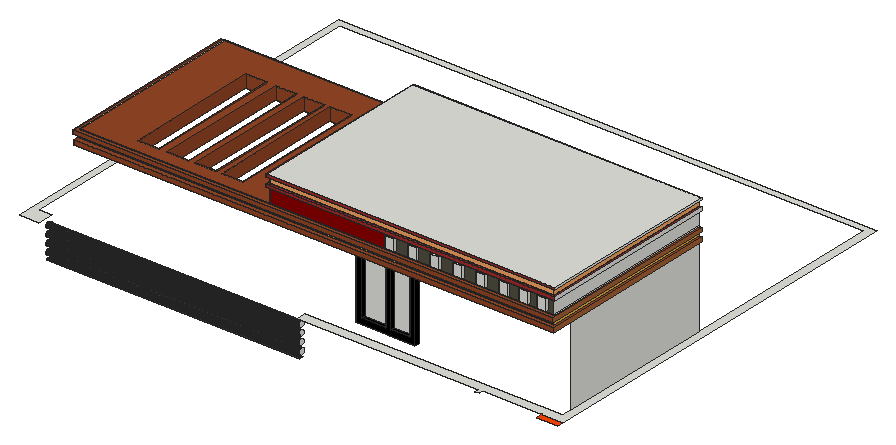
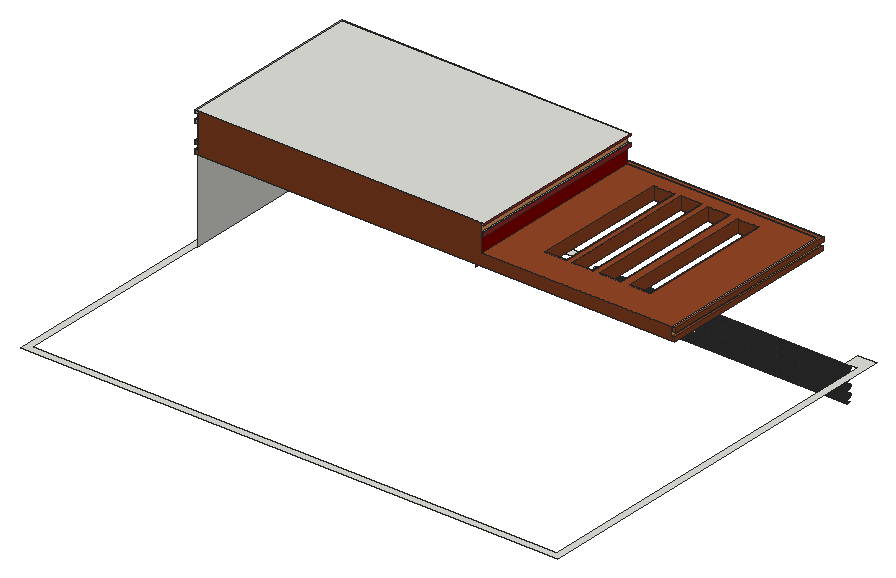
# SketchUp Ruby script. Lengths in inches.
U = 1.inch
M = Sketchup.active_model
def pt(a) = Geom::Point3d.new(a.map { |v| v * U })
def face(e, loops, mat)
  f = e.add_face(loops[0].map { |a| pt(a) })
  loops[1..].each { |l| e.add_face(l.map { |a| pt(a) }).erase! }
  f.material = f.back_material = mat if mat
  f
end
# faces: each face lists its corners as indices into pts; further lists are holes
def faces(e, pts, list, mat = nil) = list.each { |f| face(e, (f[0].is_a?(Array) ? f : [f]).map { |l| l.map { |i| pts[i] } }, mat) }
# xy, xz, yz: faces in a plane at the given z, y or x. An outline is a flat list of corners, or four numbers for a rectangle; further outlines are holes
def ring(l) = l.size == 4 ? [[l[0], l[1]], [l[2], l[1]], [l[2], l[3]], [l[0], l[3]]] : l.each_slice(2).to_a
def flat(e, list, mat, &to3) = list.each { |f| face(e, (f[0].is_a?(Array) ? f : [f]).map { |l| ring(l).map { |u, v| to3.(u, v) } }, mat) }
def xy(e, z, list, mat = nil) = flat(e, list, mat) { |x, y| [x, y, z] }
def xz(e, y, list, mat = nil) = flat(e, list, mat) { |x, z| [x, y, z] }
def yz(e, x, list, mat = nil) = flat(e, list, mat) { |y, z| [x, y, z] }
def lines(e, pts, list) = list.each { |a, b| e.add_line(pt(pts[a]), pt(pts[b])) }
# prism: a flat outline (further loops are holes) pulled along v
def prism(e, loops, v, mat = nil)
  f = face(e, loops, mat); d = Geom::Vector3d.new(v.map { |x| x * U })
  f.pushpull(f.normal.samedirection?(d) ? d.length : -d.length)
end
def box(e, o, s, mat = nil) = prism(e, [[o, [o[0] + s[0], o[1], o[2]], [o[0] + s[0], o[1] + s[1], o[2]], [o[0], o[1] + s[1], o[2]]]], [0, 0, s[2]], mat)
def at(x, y, z, deg = 0) = Geom::Transformation.translation(pt([x, y, z])) * Geom::Transformation.rotation(ORIGIN, Z_AXIS, deg.degrees)
def axes(o, x, y, z) = Geom::Transformation.new([*x, 0, *y, 0, *z, 0, *pt(o).to_a, 1])
def part(name) = M.definitions.add(name)
# library, detail: a bought-in or finely detailed component or shape, given as its bounding box
def library(name, o, s) = part(name).tap { |d| box(d.entities, o, s) }
def detail(e, o, s) = box(e.add_group.entities, o, s)
def put(e, d, t, mat = nil) = e.add_instance(d, t).tap { |i| i.material = mat if mat }
def group(e, t, mat = nil) = e.add_group.tap { |g| g.transformation = t; g.material = mat if mat }.entities
root = M.entities
M.materials.add("[0018_Brown]").color = [165, 42, 42]
M.materials.add("[0020_Red]").color = [255, 0, 0]
M.materials.add("[0021_DarkRed]").color = [139, 0, 0]
M.materials.add("[0024_OrangeRed]").color = [255, 69, 0]
M.materials.add("[0035_Tan]").color = [232, 181, 59]
M.materials.add("[0037_SandyBrown]").color = [244, 164, 96]
M.materials.add("[0137_Black]").color = [0, 0, 0]
M.materials.add("[Asphalt New]").color = [67, 60, 62]
M.materials.add("[Stone Coursed Rough]1").color = [81, 79, 64]
M.materials.add("[Wood Veneer 01]").color = [147, 70, 37]
M.materials.add("[Wood Veneer 01]1").color = [165, 96, 51]
xy(root,437.16,[[408.85,294.98,489.23,300.98]],"[0137_Black]")
xy(root,444.75,[[416.4375,294.98,449.04,300.98],[455.68,294.98,481.64,300.98]],"[0137_Black]")
xy(root,450,[[0,236.25,25.71,236.25,25.71,257.25,9,257.25,9,767.8125,720.125,767.8125,720.125,257.25,369.99,257.25,369.99,245.125,615.29,245.125,615.29,239.125,621.57,239.125,621.57,245.125,730.1875,245.125,730.1875,776.8125,0,776.8125]])
xy(root,450,[[701.81,236.125,730.1875,245.125]],"[0024_OrangeRed]")
xy(root,528.07,[[416.4375,294.98,449.04,300.98],[455.68,294.98,481.64,300.98]],"[0137_Black]")
xy(root,535.66,[[408.85,294.98,489.23,300.98]],"[0137_Black]")
xy(root,561.0625,[[706.26,270.98,706.26,294.98,507.58,294.98,507.58,300.98,720.125,300.98,720.125,270.98],[99.47,293.9,132.15,300.98],[99.47,300.98,132.15,318.33]])
xy(root,561.0625,[[[72.09,236.23,72.09,488.35,342.3125,488.35,342.3125,300.98,507.58,300.98,507.58,294.98,706.26,294.98,706.26,270.98,720.125,270.98,720.125,488.35,724.125,488.35,724.125,236.23],[253.17,261.42,281.98,445.86],[217.23,261.42,246.04,445.86],[179.29,261.42,208.11,445.86],[138.98,261.42,167.79,445.86],[99.47,293.9,132.15,318.33]]],"[Wood Veneer 01]")
xy(root,567.18,[[72.09,236.23,724.125,236.23,724.125,488.35,720.125,488.35,720.125,242.23,75.53,242.23,75.53,488.35,72.09,488.35]],"[Wood Veneer 01]")
xy(root,573.3,[[71.28,236.23,71.28,488.35,75.53,488.35,75.53,242.23,720.125,242.23,720.125,488.35,723.75,488.35,723.75,236.23]],"[Wood Veneer 01]")
xy(root,578.4375,[[71.28,236.23,723.75,236.23,723.75,488.35,720.125,488.35,720.125,242.23,75.53,242.23,75.53,488.35,71.28,488.35],[[75.53,242.23,333.59,488.35],[179.29,261.42,208.11,445.86],[217.23,261.42,246.04,445.86],[253.17,261.42,281.98,445.86],[138.98,261.42,167.79,445.86]]],"[Wood Veneer 01]")
xy(root,581.12,[[492.41,239.23,504.66,242.23],[523.34,239.23,535.59,242.23],[554.28,239.23,566.53,242.23],[585.22,239.23,597.47,242.23],[616.16,239.23,628.41,242.23],
  [647.09,239.23,659.34,242.23],[674.53,239.23,686.78,242.23],[698.84,239.23,711.09,242.23]])
xy(root,596.49,[[492.41,239.23,504.66,242.23],[523.34,239.23,535.59,242.23],[554.28,239.23,566.53,242.23],[585.22,239.23,597.47,242.23],[616.16,239.23,628.41,242.23],
  [647.09,239.23,659.34,242.23],[674.53,239.23,686.78,242.23],[698.84,239.23,711.09,242.23]])
xy(root,598.8125,[[330.96,239.23,330.96,488.35,333.59,488.35,333.59,242.23,720.125,242.23,720.125,488.35,724.125,488.35,724.125,239.23]],"[0018_Brown]")
xy(root,603.39,[[330.96,239.23,724.125,239.23,724.125,488.35,720.125,488.35,720.125,242.23,333.59,242.23,333.59,488.35,330.96,488.35]],"[0018_Brown]")
xy(root,611.61,[[330.96,239.23,330.96,488.35,333.59,488.35,333.59,242.23,720.125,242.23,720.125,488.35,723.625,488.35,723.625,239.23]],"[0018_Brown]")
xy(root,614.4375,[[330.96,239.23,723.625,488.35]])
xz(root,236.23,[[72.09,561.0625,724.125,567.18],[71.28,573.3,723.75,578.4375]],"[Wood Veneer 01]")
xz(root,239.23,[[492.41,581.12,504.66,596.49],[523.34,581.12,535.59,596.49],[554.28,581.12,566.53,596.49],[585.22,581.12,597.47,596.49],[616.16,581.12,628.41,596.49],
  [647.09,581.12,659.34,596.49],[674.53,581.12,686.78,596.49],[698.84,581.12,711.09,596.49]])
xz(root,239.23,[[330.96,598.8125,724.125,603.39],[330.96,611.61,723.625,614.4375]],"[0018_Brown]")
xz(root,242.23,[[75.53,573.3,720.125,578.4375],[333.59,598.8125,720.125,603.39]])
xz(root,242.23,[[333.59,578.4375,491.23,598.8125]],"[0021_DarkRed]")
xz(root,242.23,[[75.53,567.18,720.125,573.3]],"[0035_Tan]")
xz(root,242.23,[[333.59,603.39,720.125,611.61]],"[0037_SandyBrown]")
xz(root,242.23,[[[491.23,578.4375,720.125,598.8125],[698.84,581.12,711.09,596.49],[674.53,581.12,686.78,596.49],[647.09,581.12,659.34,596.49],[616.16,581.12,628.41,596.49],[585.22,581.12,597.47,596.49],[554.28,581.12,566.53,596.49],[523.34,581.12,535.59,596.49],[492.41,581.12,504.66,596.49]]],"[Stone Coursed Rough]1")
xz(root,261.42,[[138.98,561.0625,167.79,578.4375],[179.29,561.0625,208.11,578.4375],[217.23,561.0625,246.04,578.4375],[253.17,561.0625,281.98,578.4375]],"[Wood Veneer 01]")
xz(root,294.98,[[[408.85,437.16,489.23,535.66],[416.4375,444.75,449.04,528.07],[455.68,444.75,481.64,528.07]]],"[0137_Black]")
xz(root,300.98,[[416.4375,444.75,449.04,528.07],[455.68,444.75,481.64,528.07]])
xz(root,445.86,[[138.98,561.0625,167.79,578.4375],[179.29,561.0625,208.11,578.4375],[217.23,561.0625,246.04,578.4375],[253.17,561.0625,281.98,578.4375]],"[Wood Veneer 01]")
xz(root,488.35,[[330.96,598.8125,333.59,603.39],[720.125,598.8125,724.125,603.39],[330.96,611.61,333.59,614.4375],[720.125,611.61,723.625,614.4375]])
xz(root,488.35,[[75.53,561.0625,75.53,578.4375,333.59,578.4375,333.59,614.4375,720.125,614.4375,720.125,561.0625]],"[Wood Veneer 01]")
xz(root,488.35,[[72.09,561.0625,75.53,567.18],[720.125,561.0625,724.125,567.18],[71.28,573.3,75.53,578.4375],[720.125,573.3,723.75,578.4375]],"[Wood Veneer 01]1")
yz(root,71.28,[[236.23,573.3,488.35,578.4375]],"[Wood Veneer 01]")
yz(root,72.09,[[236.23,561.0625,488.35,567.18]],"[Wood Veneer 01]")
yz(root,75.53,[[242.23,573.3,488.35,578.4375]])
yz(root,75.53,[[242.23,567.18,488.35,573.3]],"[0035_Tan]")
yz(root,99.47,[[300.98,561.0625,318.33,562.9375]])
yz(root,138.98,[[261.42,561.0625,445.86,578.4375]],"[Wood Veneer 01]")
yz(root,167.79,[[261.42,561.0625,445.86,578.4375]],"[Wood Veneer 01]")
yz(root,179.29,[[261.42,561.0625,445.86,578.4375]],"[Wood Veneer 01]")
yz(root,208.11,[[261.42,561.0625,445.86,578.4375]],"[Wood Veneer 01]")
yz(root,217.23,[[261.42,561.0625,445.86,578.4375]],"[Wood Veneer 01]")
yz(root,246.04,[[261.42,561.0625,445.86,578.4375]],"[Wood Veneer 01]")
yz(root,253.17,[[261.42,561.0625,445.86,578.4375]],"[Wood Veneer 01]")
yz(root,281.98,[[261.42,561.0625,445.86,578.4375]],"[Wood Veneer 01]")
yz(root,330.96,[[239.23,598.8125,488.35,603.39],[239.23,611.61,488.35,614.4375]],"[0018_Brown]")
yz(root,333.59,[[242.23,598.8125,488.35,603.39]])
yz(root,333.59,[[242.23,578.4375,488.35,598.8125]],"[0021_DarkRed]")
yz(root,333.59,[[242.23,603.39,488.35,611.61]],"[0037_SandyBrown]")
yz(root,342.3125,[[300.98,557.75,488.35,561.0625]],"[0020_Red]")
yz(root,369.99,[[251.48,414.82,252.42,414.95,253.3,415.31,254.05,415.89,254.62,416.64,254.98,417.51,255.11,418.45,254.98,419.39,254.62,420.26,254.05,421.01,253.3,421.59,252.42,421.95,251.48,422.07,250.54,421.95,249.67,421.59,248.92,421.01,248.34,420.26,248.25,420.04,248.25,416.86,248.34,416.64,248.92,415.89,249.67,415.31,250.54,414.95],[248.25,416.86,247.98,417.51,247.86,418.45,247.98,419.39,248.25,420.04],[251.48,425.76,252.42,425.89,253.3,426.25,254.05,426.82,254.62,427.57,254.98,428.45,255.11,429.39,254.98,430.33,254.62,431.2,254.05,431.95,253.3,432.53,252.42,432.89,251.48,433.01,250.54,432.89,249.67,432.53,248.92,431.95,248.34,431.2,248.25,430.97,248.25,427.8,248.34,427.57,248.92,426.82,249.67,426.25,250.54,425.89],[248.25,427.8,247.98,428.45,247.86,429.39,247.98,430.33,248.25,430.97],[251.48,436.7,252.42,436.82,253.3,437.19,254.05,437.76,254.62,438.51,254.98,439.39,255.11,440.32,254.98,441.26,254.62,442.14,254.05,442.89,253.3,443.46,252.42,443.83,251.48,443.95,250.54,443.83,249.67,443.46,248.92,442.89,248.34,442.14,248.25,441.91,248.25,438.74,248.34,438.51,248.92,437.76,249.67,437.19,250.54,436.82],
  [248.25,438.74,247.98,439.39,247.86,440.32,247.98,441.26,248.25,441.91]])
yz(root,370.39,[[251.48,403.89,252.42,404.01,253.3,404.37,254.05,404.95,254.62,405.7,254.98,406.57,255.11,407.51,254.98,408.45,254.62,409.32,254.05,410.08,253.3,410.65,252.42,411.01,251.48,411.14,250.54,411.01,249.67,410.65,248.92,410.08,248.34,409.32,247.98,408.45,247.86,407.51,247.98,406.57,248.34,405.7,248.92,404.95,249.67,404.37,250.54,404.01]])
yz(root,408.85,[[294.98,437.16,300.98,535.66]],"[0137_Black]")
yz(root,416.4375,[[294.98,444.75,300.98,528.07]],"[0137_Black]")
yz(root,449.04,[[294.98,444.75,300.98,528.07]],"[0137_Black]")
yz(root,455.68,[[294.98,444.75,300.98,528.07]],"[0137_Black]")
yz(root,481.64,[[294.98,444.75,300.98,528.07]],"[0137_Black]")
yz(root,489.23,[[294.98,437.16,300.98,535.66]],"[0137_Black]")
yz(root,492.41,[[239.23,581.12,242.23,596.49]])
yz(root,504.66,[[239.23,581.12,242.23,596.49]])
yz(root,523.34,[[239.23,581.12,242.23,596.49]])
yz(root,535.59,[[239.23,581.12,242.23,596.49]])
yz(root,554.28,[[239.23,581.12,242.23,596.49]])
yz(root,566.53,[[239.23,581.12,242.23,596.49]])
yz(root,585.22,[[239.23,581.12,242.23,596.49]])
yz(root,597.47,[[239.23,581.12,242.23,596.49]])
yz(root,616.16,[[239.23,581.12,242.23,596.49]])
yz(root,628.41,[[239.23,581.12,242.23,596.49]])
yz(root,647.09,[[239.23,581.12,242.23,596.49]])
yz(root,659.34,[[239.23,581.12,242.23,596.49]])
yz(root,674.53,[[239.23,581.12,242.23,596.49]])
yz(root,686.78,[[239.23,581.12,242.23,596.49]])
yz(root,698.84,[[239.23,581.12,242.23,596.49]])
yz(root,711.09,[[239.23,581.12,242.23,596.49]])
yz(root,720.125,[[270.98,450,488.35,561.0625],[242.23,573.3,488.35,578.4375],[242.23,578.4375,488.35,598.8125],[242.23,598.8125,488.35,603.39]])
yz(root,720.125,[[242.23,567.18,488.35,573.3]],"[0035_Tan]")
yz(root,720.125,[[242.23,603.39,488.35,611.61]],"[0037_SandyBrown]")
yz(root,723.625,[[239.23,611.61,488.35,614.4375]])
yz(root,723.75,[[236.23,573.3,488.35,578.4375]],"[Wood Veneer 01]1")
yz(root,724.125,[[239.23,598.8125,488.35,603.39]])
yz(root,724.125,[[236.23,561.0625,488.35,567.18]],"[Wood Veneer 01]1")
p = [[25.71,249.67,399.71],[25.71,248.92,399.14],[369.99,248.92,399.14],[369.99,249.67,399.71],[25.71,254.05,399.14],[25.71,253.3,399.71],
  [369.99,253.3,399.71],[369.99,254.05,399.14],[25.71,250.54,400.08],[369.99,250.54,400.08],[25.71,252.42,400.08],[369.99,252.42,400.08],
  [25.71,251.48,400.2],[369.99,251.48,400.2],[25.71,250.54,404.01],[25.71,251.48,403.89],[370.39,251.48,403.89],[370.39,250.54,404.01],
  [25.71,252.42,404.01],[370.39,252.42,404.01],[25.71,249.67,404.37],[370.39,249.67,404.37],[25.71,253.3,404.37],[370.39,253.3,404.37],
  [25.71,248.92,404.95],[370.39,248.92,404.95],[25.71,254.05,404.95],[370.39,254.05,404.95],[25.71,248.34,405.7],[370.39,248.34,405.7],
  [25.71,254.62,405.7],[370.39,254.62,405.7],[25.71,247.98,406.57],[370.39,247.98,406.57],[25.71,254.98,406.57],[370.39,254.98,406.57],
  [25.71,247.86,407.51],[370.39,247.86,407.51],[25.71,255.11,407.51],[370.39,255.11,407.51],[25.71,247.98,408.45],[370.39,247.98,408.45],
  [25.71,254.98,408.45],[370.39,254.98,408.45],[25.71,248.34,409.32],[370.39,248.34,409.32],[25.71,254.62,409.32],[370.39,254.62,409.32],
  [25.71,248.92,410.08],[370.39,248.92,410.08],[25.71,254.05,410.08],[370.39,254.05,410.08],[25.71,249.67,410.65],[370.39,249.67,410.65],
  [25.71,253.3,410.65],[370.39,253.3,410.65],[25.71,250.54,411.01],[370.39,250.54,411.01],[25.71,252.42,411.01],[370.39,252.42,411.01],
  [25.71,251.48,411.14],[370.39,251.48,411.14],[25.71,250.54,414.95],[25.71,251.48,414.82],[369.99,251.48,414.82],[369.99,250.54,414.95],
  [25.71,252.42,414.95],[369.99,252.42,414.95],[25.71,249.67,415.31],[369.99,249.67,415.31],[25.71,253.3,415.31],[369.99,253.3,415.31],
  [25.71,248.92,415.89],[369.99,248.92,415.89],[25.71,254.05,415.89],[369.99,254.05,415.89],[25.71,248.34,416.64],[369.99,248.34,416.64],
  [25.71,254.62,416.64],[369.99,254.62,416.64],[25.71,247.98,417.51],[369.99,248.25,416.86],[369.99,247.98,417.51],[25.71,254.98,417.51],
  [369.99,254.98,417.51],[25.71,247.86,418.45],[369.99,247.86,418.45],[25.71,255.11,418.45],[369.99,255.11,418.45],[25.71,247.98,419.39],
  [369.99,247.98,419.39],[25.71,254.98,419.39],[369.99,254.98,419.39],[25.71,248.34,420.26],[369.99,248.25,420.04],[369.99,248.34,420.26],
  [25.71,254.62,420.26],[369.99,254.62,420.26],[25.71,248.92,421.01],[369.99,248.92,421.01],[25.71,254.05,421.01],[369.99,254.05,421.01],
  [25.71,249.67,421.59],[369.99,249.67,421.59],[25.71,253.3,421.59],[369.99,253.3,421.59],[25.71,250.54,421.95],[369.99,250.54,421.95],
  [25.71,252.42,421.95],[369.99,252.42,421.95],[25.71,251.48,422.07],[369.99,251.48,422.07],[25.71,250.54,425.89],[25.71,251.48,425.76],
  [369.99,251.48,425.76],[369.99,250.54,425.89],[25.71,252.42,425.89],[369.99,252.42,425.89],[25.71,249.67,426.25],[369.99,249.67,426.25],
  [25.71,253.3,426.25],[369.99,253.3,426.25],[25.71,248.92,426.82],[369.99,248.92,426.82],[25.71,254.05,426.82],[369.99,254.05,426.82],
  [25.71,248.34,427.57],[369.99,248.34,427.57],[25.71,254.62,427.57],[369.99,254.62,427.57],[25.71,247.98,428.45],[369.99,248.25,427.8],
  [369.99,247.98,428.45],[25.71,254.98,428.45],[369.99,254.98,428.45],[25.71,247.86,429.39],[369.99,247.86,429.39],[25.71,255.11,429.39],
  [369.99,255.11,429.39],[25.71,247.98,430.33],[369.99,247.98,430.33],[25.71,254.98,430.33],[369.99,254.98,430.33],[25.71,248.34,431.2],
  [369.99,248.25,430.97],[369.99,248.34,431.2],[25.71,254.62,431.2],[369.99,254.62,431.2],[25.71,248.92,431.95],[369.99,248.92,431.95],
  [25.71,254.05,431.95],[369.99,254.05,431.95],[25.71,249.67,432.53],[369.99,249.67,432.53],[25.71,253.3,432.53],[369.99,253.3,432.53],
  [25.71,250.54,432.89],[369.99,250.54,432.89],[25.71,252.42,432.89],[369.99,252.42,432.89],[25.71,251.48,433.01],[369.99,251.48,433.01],
  [25.71,250.54,436.82],[25.71,251.48,436.7],[369.99,251.48,436.7],[369.99,250.54,436.82],[25.71,252.42,436.82],[369.99,252.42,436.82],
  [25.71,249.67,437.19],[369.99,249.67,437.19],[25.71,253.3,437.19],[369.99,253.3,437.19],[25.71,248.92,437.76],[369.99,248.92,437.76],
  [25.71,254.05,437.76],[369.99,254.05,437.76],[25.71,248.34,438.51],[369.99,248.34,438.51],[25.71,254.62,438.51],[369.99,254.62,438.51],
  [25.71,247.98,439.39],[369.99,248.25,438.74],[369.99,247.98,439.39],[25.71,254.98,439.39],[369.99,254.98,439.39],[25.71,247.86,440.32],
  [369.99,247.86,440.32],[25.71,255.11,440.32],[369.99,255.11,440.32],[25.71,247.98,441.26],[369.99,247.98,441.26],[25.71,254.98,441.26],
  [369.99,254.98,441.26],[25.71,248.34,442.14],[369.99,248.25,441.91],[369.99,248.34,442.14],[25.71,254.62,442.14],[369.99,254.62,442.14],
  [25.71,248.92,442.89],[369.99,248.92,442.89],[25.71,254.05,442.89],[369.99,254.05,442.89],[25.71,249.67,443.46],[369.99,249.67,443.46],
  [25.71,253.3,443.46],[369.99,253.3,443.46],[25.71,250.54,443.83],[369.99,250.54,443.83],[25.71,252.42,443.83],[369.99,252.42,443.83],
  [25.71,251.48,443.95],[369.99,251.48,443.95],[99.47,488.35,562.9375],[99.47,318.33,562.9375],[76.59,300.98,561.0625],[76.59,300.98,563.5],
  [76.59,282.66,563.5],[75.53,300.98,563.5],[720.125,242.23,561.0625],[720.125,242.23,567.18],[75.53,242.23,561.0625],[75.53,242.23,567.18],
  [720.125,242.23,611.61],[720.125,242.23,614.4375]]
faces(root,p,[[0,1,2,3],[4,5,6,7],[8,0,3,9],[5,10,11,6],[12,8,9,13],[10,12,13,11],[14,15,16,17],[15,18,19,16],
  [20,14,17,21],[18,22,23,19],[24,20,21,25],[22,26,27,23],[28,24,25,29],[26,30,31,27],[32,28,29,33],[30,34,35,31],
  [36,32,33,37],[34,38,39,35],[40,36,37,41],[38,42,43,39],[44,40,41,45],[42,46,47,43],[48,44,45,49],[46,50,51,47],
  [52,48,49,53],[50,54,55,51],[56,52,53,57],[54,58,59,55],[60,56,57,61],[58,60,61,59],[62,63,64,65],[63,66,67,64],
  [68,62,65,69],[66,70,71,67],[72,68,69,73],[70,74,75,71],[76,72,73,77],[74,78,79,75],[80,76,77,81,82],[78,83,84,79],
  [85,80,82,86],[83,87,88,84],[89,85,86,90],[87,91,92,88],[93,89,90,94,95],[91,96,97,92],[98,93,95,99],[96,100,101,97],
  [102,98,99,103],[100,104,105,101],[106,102,103,107],[104,108,109,105],[110,106,107,111],[108,110,111,109],[112,113,114,115],[113,116,117,114],
  [118,112,115,119],[116,120,121,117],[122,118,119,123],[120,124,125,121],[126,122,123,127],[124,128,129,125],[130,126,127,131,132],[128,133,134,129],
  [135,130,132,136],[133,137,138,134],[139,135,136,140],[137,141,142,138],[143,139,140,144,145],[141,146,147,142],[148,143,145,149],[146,150,151,147],
  [152,148,149,153],[150,154,155,151],[156,152,153,157],[154,158,159,155],[160,156,157,161],[158,160,161,159],[162,163,164,165],[163,166,167,164],
  [168,162,165,169],[166,170,171,167],[172,168,169,173],[170,174,175,171],[176,172,173,177],[174,178,179,175],[180,176,177,181,182],[178,183,184,179],
  [185,180,182,186],[183,187,188,184],[189,185,186,190],[187,191,192,188],[193,189,190,194,195],[191,196,197,192],[198,193,195,199],[196,200,201,197],
  [202,198,199,203],[200,204,205,201],[206,202,203,207],[204,208,209,205],[210,206,207,211],[208,210,211,209]],"[Asphalt New]")
lines(root,p,[[212,213],[214,215],[215,216],[217,215],[218,219],[220,221],[222,223]])
